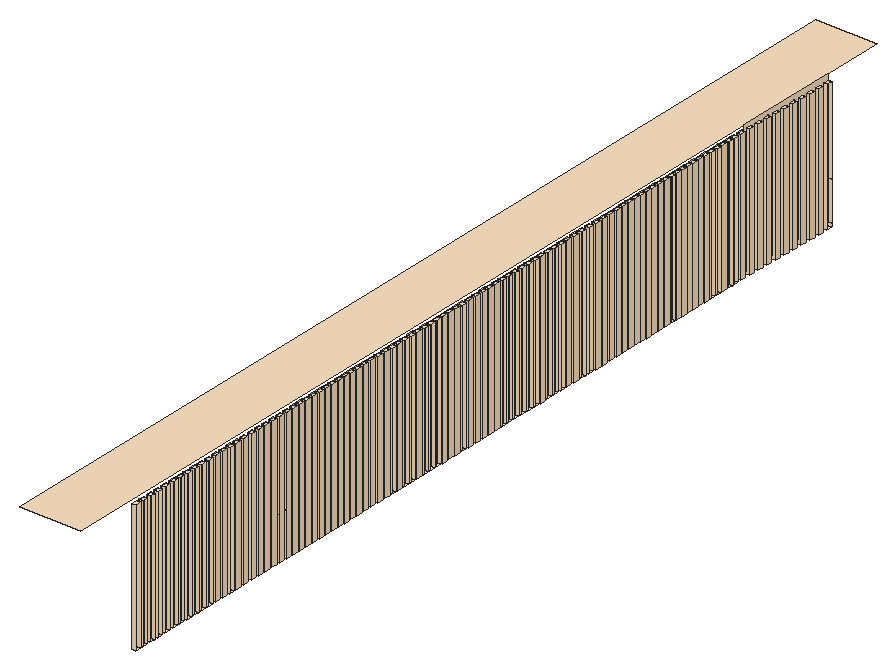
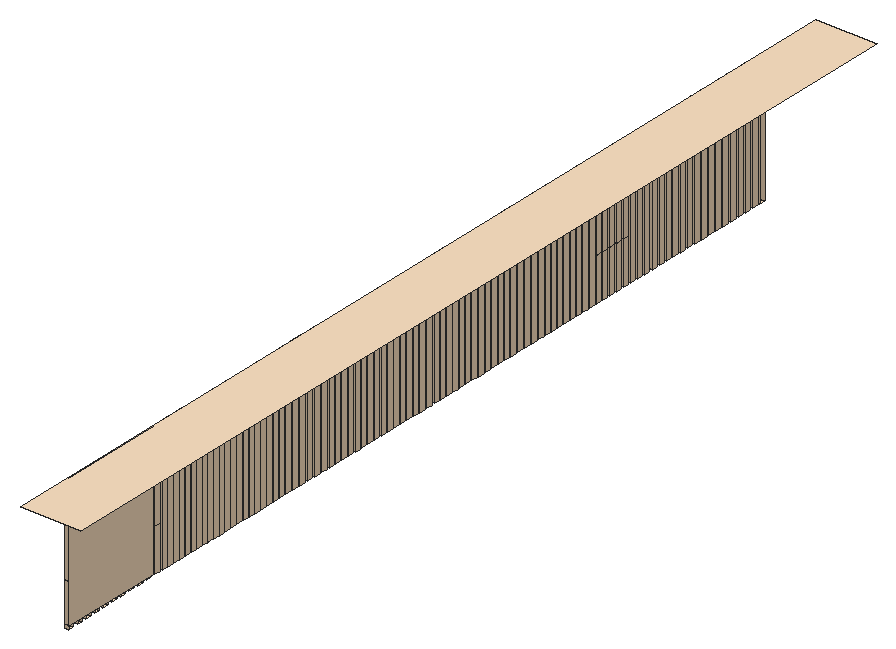
# SketchUp Ruby script. Lengths in inches.
U = 1.inch
M = Sketchup.active_model
def pt(a) = Geom::Point3d.new(a.map { |v| v * U })
def face(e, loops, mat)
  f = e.add_face(loops[0].map { |a| pt(a) })
  loops[1..].each { |l| e.add_face(l.map { |a| pt(a) }).erase! }
  f.material = f.back_material = mat if mat
  f
end
# faces: each face lists its corners as indices into pts; further lists are holes
def faces(e, pts, list, mat = nil) = list.each { |f| face(e, (f[0].is_a?(Array) ? f : [f]).map { |l| l.map { |i| pts[i] } }, mat) }
# xy, xz, yz: faces in a plane at the given z, y or x. An outline is a flat list of corners, or four numbers for a rectangle; further outlines are holes
def ring(l) = l.size == 4 ? [[l[0], l[1]], [l[2], l[1]], [l[2], l[3]], [l[0], l[3]]] : l.each_slice(2).to_a
def flat(e, list, mat, &to3) = list.each { |f| face(e, (f[0].is_a?(Array) ? f : [f]).map { |l| ring(l).map { |u, v| to3.(u, v) } }, mat) }
def xy(e, z, list, mat = nil) = flat(e, list, mat) { |x, y| [x, y, z] }
def xz(e, y, list, mat = nil) = flat(e, list, mat) { |x, z| [x, y, z] }
def yz(e, x, list, mat = nil) = flat(e, list, mat) { |y, z| [x, y, z] }
def lines(e, pts, list) = list.each { |a, b| e.add_line(pt(pts[a]), pt(pts[b])) }
# prism: a flat outline (further loops are holes) pulled along v
def prism(e, loops, v, mat = nil)
  f = face(e, loops, mat); d = Geom::Vector3d.new(v.map { |x| x * U })
  f.pushpull(f.normal.samedirection?(d) ? d.length : -d.length)
end
def box(e, o, s, mat = nil) = prism(e, [[o, [o[0] + s[0], o[1], o[2]], [o[0] + s[0], o[1] + s[1], o[2]], [o[0], o[1] + s[1], o[2]]]], [0, 0, s[2]], mat)
def at(x, y, z, deg = 0) = Geom::Transformation.translation(pt([x, y, z])) * Geom::Transformation.rotation(ORIGIN, Z_AXIS, deg.degrees)
def axes(o, x, y, z) = Geom::Transformation.new([*x, 0, *y, 0, *z, 0, *pt(o).to_a, 1])
def part(name) = M.definitions.add(name)
# library, detail: a bought-in or finely detailed component or shape, given as its bounding box
def library(name, o, s) = part(name).tap { |d| box(d.entities, o, s) }
def detail(e, o, s) = box(e.add_group.entities, o, s)
def put(e, d, t, mat = nil) = e.add_instance(d, t).tap { |i| i.material = mat if mat }
def group(e, t, mat = nil) = e.add_group.tap { |g| g.transformation = t; g.material = mat if mat }.entities
root = M.entities
M.materials.add("[0012_Bisque]").color = [255, 228, 196]
box(root,[9,118.66,100.0625],[0.5625,0.83,19.4375],"[0012_Bisque]")
box(root,[9,119.72,100.0625],[0.5625,0.83,19.4375],"[0012_Bisque]")
box(root,[9,100.09,100.0625],[0.5625,0.83,19.4375],"[0012_Bisque]")
box(root,[9,63.78,100.0625],[0.5625,0.83,19.4375],"[0012_Bisque]")
box(root,[9,126.29,100.0625],[0.5625,0.83,19.4375],"[0012_Bisque]")
box(root,[9,125.29,100.0625],[0.5625,0.83,19.4375],"[0012_Bisque]")
box(root,[9,77.21,100.0625],[0.5625,0.84,19.4375],"[0012_Bisque]")
box(root,[9,81.96,100.0625],[0.5625,0.84,19.4375],"[0012_Bisque]")
box(root,[9,84.28,100.0625],[0.5625,0.83,19.4375],"[0012_Bisque]")
box(root,[9,88.09,100.0625],[0.5625,0.83,19.4375],"[0012_Bisque]")
box(root,[9,86.78,100.0625],[0.5625,0.83,19.4375],"[0012_Bisque]")
box(root,[9,121.97,100.125],[0.5625,0.83,19.375],"[0012_Bisque]")
box(root,[9,106.28,100.125],[0.5625,0.83,19.375],"[0012_Bisque]")
box(root,[9,104.9,100.125],[0.5625,0.83,19.375],"[0012_Bisque]")
box(root,[9,130.47,100.125],[0.5625,0.83,19.375],"[0012_Bisque]")
box(root,[9,127.35,100.125],[0.5625,0.83,19.375],"[0012_Bisque]")
box(root,[9,129.41,100.125],[0.5625,0.83,19.375],"[0012_Bisque]")
box(root,[9,133.72,100.125],[0.5625,0.83,19.375],"[0012_Bisque]")
box(root,[9,120.79,100.125],[0.5625,0.83,19.375],"[0012_Bisque]")
box(root,[9,123.16,100.125],[0.5625,0.83,19.375],"[0012_Bisque]")
box(root,[9,115.29,100.125],[0.5625,0.83,19.375],"[0012_Bisque]")
box(root,[9,89.34,100.125],[0.5625,0.83,19.375],"[0012_Bisque]")
box(root,[9,116.47,100.125],[0.5625,0.83,19.375],"[0012_Bisque]")
box(root,[9,117.6,100.125],[0.5625,0.83,19.375],"[0012_Bisque]")
box(root,[9,66.09,100.125],[0.5625,0.83,19.375],"[0012_Bisque]")
box(root,[9,64.9,100.125],[0.5625,0.83,19.375],"[0012_Bisque]")
box(root,[9,69.96,100.125],[0.5625,0.84,19.375],"[0012_Bisque]")
box(root,[9,68.65,100.125],[0.5625,0.83,19.375],"[0012_Bisque]")
box(root,[9,67.34,100.125],[0.5625,0.83,19.375],"[0012_Bisque]")
box(root,[9,73.59,100.125],[0.5625,0.83,19.375],"[0012_Bisque]")
box(root,[9,43.71,100.125],[0.5625,0.84,19.375],"[0012_Bisque]")
box(root,[9,47.84,100.125],[0.5625,0.83,19.375],"[0012_Bisque]")
box(root,[9,39.9,100.125],[0.5625,0.83,19.375],"[0012_Bisque]")
box(root,[9,46.53,100.125],[0.5625,0.83,19.375],"[0012_Bisque]")
box(root,[9,57.9,100.125],[0.5625,0.83,19.375],"[0012_Bisque]")
box(root,[9,60.28,100.125],[0.5625,0.83,19.375],"[0012_Bisque]")
box(root,[9,61.46,100.125],[0.5625,0.84,19.375],"[0012_Bisque]")
box(root,[9,49.09,100.125],[0.5625,0.83,19.375],"[0012_Bisque]")
box(root,[9,71.28,100.125],[0.5625,0.83,19.375],"[0012_Bisque]")
box(root,[9,41.21,100.125],[0.5625,0.84,19.375],"[0012_Bisque]")
box(root,[9,56.65,100.125],[0.5625,0.83,19.375],"[0012_Bisque]")
box(root,[9,45.09,100.125],[0.5625,0.83,19.375],"[0012_Bisque]")
box(root,[9,59.15,100.125],[0.5625,0.83,19.375],"[0012_Bisque]")
box(root,[9,83.15,100.125],[0.5625,0.83,19.375],"[0012_Bisque]")
box(root,[9,91.71,100.125],[0.5625,0.84,19.375],"[0012_Bisque]")
box(root,[9,128.35,100.125],[0.5625,0.83,19.375],"[0012_Bisque]")
box(root,[9,90.53,100.125],[0.5625,0.83,19.375],"[0012_Bisque]")
box(root,[9,62.65,100.125],[0.5625,0.83,19.375],"[0012_Bisque]")
box(root,[9.0625,110.28,100.0625],[0.5625,0.83,19.4375],"[0012_Bisque]")
box(root,[9.0625,111.53,100.0625],[0.5625,0.83,19.4375],"[0012_Bisque]")
box(root,[9.0625,114.09,100.125],[0.5625,0.83,19.375],"[0012_Bisque]")
box(root,[9.0625,112.84,100.125],[0.5625,0.83,19.375],"[0012_Bisque]")
xy(root,99.78,[[9.03,153.16,9.59,154]],"[0012_Bisque]")
xy(root,99.8125,[[9.02,151.56,9.59,152.4]],"[0012_Bisque]")
xy(root,99.85,[[9.02,149.96,9.58,150.8]],"[0012_Bisque]")
xy(root,99.88,[[9.02,148.37,9.58,149.2]],"[0012_Bisque]")
xy(root,99.92,[[9.02,146.77,9.58,147.6]],"[0012_Bisque]")
xy(root,99.95,[[9.01,145.17,9.58,146]],"[0012_Bisque]")
xy(root,99.99,[[9.01,143.57,9.57,144.4]],"[0012_Bisque]")
xy(root,100.02,[[9.01,141.97,9.57,142.8]],"[0012_Bisque]")
xy(root,100.06,[[9.01,140.37,9.57,141.2]],"[0012_Bisque]")
xy(root,100.09,[[9,138.77,9.57,139.6]],"[0012_Bisque]")
xy(root,100.125,[[9,25.15,9.5625,25.98],[9,26.4,9.5625,27.23],[9,27.78,9.5625,28.61],[9,29.15,9.5625,29.98],[9,30.53,9.5625,31.36],
  [9,32.03,9.5625,32.86],[9,33.28,9.5625,34.11],[9,34.59,9.5625,35.42],[9,35.9,9.5625,36.73],[9,37.21,9.5625,38.05],
  [9,38.53,9.5625,39.36],[9,42.46,9.5625,43.3],[9,50.4,9.5625,51.23],[9,51.71,9.5625,52.55],[9,53.03,9.5625,53.86],
  [9,54.28,9.5625,55.11],[9,55.46,9.5625,56.3],[9,72.46,9.5625,73.3],[9,74.78,9.5625,75.61],[9,76.03,9.5625,76.86],
  [9,78.46,9.5625,79.3],[9,79.65,9.5625,80.48],[9,80.78,9.5625,81.61],[9,85.46,9.5625,86.3],[9,92.9,9.5625,93.73],
  [9,94.03,9.5625,94.86],[9,95.21,9.5625,96.05],[9,96.53,9.5625,97.36],[9,97.78,9.5625,98.61],[9,98.96,9.5625,99.8],
  [9,101.34,9.5625,102.17],[9,102.53,9.5625,103.36],[9,103.78,9.5625,104.61],[9,107.59,9.5625,108.42],[9,108.96,9.5625,109.8],
  [9,124.22,9.5625,125.05],[9,131.54,9.5625,132.37],[9,132.66,9.5625,133.49],[9,134.79,9.5625,135.62],[9,135.85,9.5625,136.68],
  [9,137.17,9.5625,138]],"[0012_Bisque]")
xy(root,119.15,[[9.03,153.16,9.59,154]],"[0012_Bisque]")
xy(root,119.1875,[[9.02,151.56,9.59,152.4]],"[0012_Bisque]")
xy(root,119.22,[[9.02,149.96,9.58,150.8]],"[0012_Bisque]")
xy(root,119.26,[[9.02,148.37,9.58,149.2]],"[0012_Bisque]")
xy(root,119.29,[[9.02,146.77,9.58,147.6]],"[0012_Bisque]")
xy(root,119.33,[[9.01,145.17,9.58,146]],"[0012_Bisque]")
xy(root,119.36,[[9.01,143.57,9.57,144.4]],"[0012_Bisque]")
xy(root,119.4,[[9.01,141.97,9.57,142.8]],"[0012_Bisque]")
xy(root,119.43,[[9.01,140.37,9.57,141.2]],"[0012_Bisque]")
xy(root,119.47,[[9,138.77,9.57,139.6]],"[0012_Bisque]")
xy(root,119.5,[[9,25.15,9.5625,25.98],[9,26.4,9.5625,27.23],[9,27.78,9.5625,28.61],[9,29.15,9.5625,29.98],[9,30.53,9.5625,31.36],
  [9,32.03,9.5625,32.86],[9,33.28,9.5625,34.11],[9,34.59,9.5625,35.42],[9,35.9,9.5625,36.73],[9,37.21,9.5625,38.05],
  [9,38.53,9.5625,39.36],[9,42.46,9.5625,43.3],[9,50.4,9.5625,51.23],[9,51.71,9.5625,52.55],[9,53.03,9.5625,53.86],
  [9,54.28,9.5625,55.11],[9,55.46,9.5625,56.3],[9,72.46,9.5625,73.3],[9,74.78,9.5625,75.61],[9,76.03,9.5625,76.86],
  [9,78.46,9.5625,79.3],[9,79.65,9.5625,80.48],[9,80.78,9.5625,81.61],[9,85.46,9.5625,86.3],[9,92.9,9.5625,93.73],
  [9,94.03,9.5625,94.86],[9,95.21,9.5625,96.05],[9,96.53,9.5625,97.36],[9,97.78,9.5625,98.61],[9,98.96,9.5625,99.8],
  [9,101.34,9.5625,102.17],[9,102.53,9.5625,103.36],[9,103.78,9.5625,104.61],[9,107.59,9.5625,108.42],[9,108.96,9.5625,109.8],
  [9,124.22,9.5625,125.05],[9,131.54,9.5625,132.37],[9,132.66,9.5625,133.49],[9,134.79,9.5625,135.62],[9,135.85,9.5625,136.68],
  [9,137.17,9.5625,138]],"[0012_Bisque]")
xy(root,120,[[9,15.65,9,162.99,0,162.99,0,15.6875]],"[0012_Bisque]")
xz(root,25.15,[[9,100.125,9.5625,119.5]],"[0012_Bisque]")
xz(root,25.98,[[9,100.125,9.5625,119.5]],"[0012_Bisque]")
xz(root,26.4,[[9,100.125,9.5625,119.5]],"[0012_Bisque]")
xz(root,27.23,[[9,100.125,9.5625,119.5]],"[0012_Bisque]")
xz(root,27.78,[[9,100.125,9.5625,119.5]],"[0012_Bisque]")
xz(root,28.61,[[9,100.125,9.5625,119.5]],"[0012_Bisque]")
xz(root,29.15,[[9,100.125,9.5625,119.5]],"[0012_Bisque]")
xz(root,29.98,[[9,100.125,9.5625,119.5]],"[0012_Bisque]")
xz(root,30.53,[[9,100.125,9.5625,119.5]],"[0012_Bisque]")
xz(root,31.36,[[9,100.125,9.5625,119.5]],"[0012_Bisque]")
xz(root,32.03,[[9,100.125,9.5625,119.5]],"[0012_Bisque]")
xz(root,32.86,[[9,100.125,9.5625,119.5]],"[0012_Bisque]")
xz(root,33.28,[[9,100.125,9.5625,119.5]],"[0012_Bisque]")
xz(root,34.11,[[9,100.125,9.5625,119.5]],"[0012_Bisque]")
xz(root,34.59,[[9,100.125,9.5625,119.5]],"[0012_Bisque]")
xz(root,35.42,[[9,100.125,9.5625,119.5]],"[0012_Bisque]")
xz(root,35.9,[[9,100.125,9.5625,119.5]],"[0012_Bisque]")
xz(root,36.73,[[9,100.125,9.5625,119.5]],"[0012_Bisque]")
xz(root,37.21,[[9,100.125,9.5625,119.5]],"[0012_Bisque]")
xz(root,38.05,[[9,100.125,9.5625,119.5]],"[0012_Bisque]")
xz(root,38.53,[[9,100.125,9.5625,119.5]],"[0012_Bisque]")
xz(root,39.36,[[9,100.125,9.5625,119.5]],"[0012_Bisque]")
xz(root,42.46,[[9,100.125,9.5625,119.5]],"[0012_Bisque]")
xz(root,43.3,[[9,100.125,9.5625,119.5]],"[0012_Bisque]")
xz(root,50.4,[[9,100.125,9.5625,106.5],[9,106.5,9.5625,119.5]],"[0012_Bisque]")
xz(root,51.23,[[9,100.125,9.5625,106.5],[9,106.5,9.5625,119.5]],"[0012_Bisque]")
xz(root,51.71,[[9,100.125,9.5625,106.5],[9,106.5,9.5625,119.5]],"[0012_Bisque]")
xz(root,52.55,[[9,100.125,9.5625,106.5],[9,106.5,9.5625,119.5]],"[0012_Bisque]")
xz(root,53.03,[[9,100.125,9.5625,106.5],[9,106.5,9.5625,119.5]],"[0012_Bisque]")
xz(root,53.86,[[9,100.125,9.5625,106.5],[9,106.5,9.5625,119.5]],"[0012_Bisque]")
xz(root,54.28,[[9,100.125,9.5625,106.5],[9,106.5,9.5625,119.5]],"[0012_Bisque]")
xz(root,55.11,[[9,100.125,9.5625,106.5],[9,106.5,9.5625,119.5]],"[0012_Bisque]")
xz(root,55.46,[[9,100.125,9.5625,106.5],[9,106.5,9.5625,119.5]],"[0012_Bisque]")
xz(root,56.3,[[9,100.125,9.5625,106.5],[9,106.5,9.5625,119.5]],"[0012_Bisque]")
xz(root,72.46,[[9,100.125,9.5625,119.5]],"[0012_Bisque]")
xz(root,73.3,[[9,100.125,9.5625,119.5]],"[0012_Bisque]")
xz(root,74.78,[[9,100.125,9.5625,119.5]],"[0012_Bisque]")
xz(root,75.61,[[9,100.125,9.5625,119.5]],"[0012_Bisque]")
xz(root,76.03,[[9,100.125,9.5625,119.5]],"[0012_Bisque]")
xz(root,76.86,[[9,100.125,9.5625,119.5]],"[0012_Bisque]")
xz(root,78.46,[[9,100.125,9.5625,119.5]],"[0012_Bisque]")
xz(root,79.3,[[9,100.125,9.5625,119.5]],"[0012_Bisque]")
xz(root,79.65,[[9,100.125,9.5625,119.5]],"[0012_Bisque]")
xz(root,80.48,[[9,100.125,9.5625,119.5]],"[0012_Bisque]")
xz(root,80.78,[[9,100.125,9.5625,119.5]],"[0012_Bisque]")
xz(root,81.61,[[9,100.125,9.5625,119.5]],"[0012_Bisque]")
xz(root,85.46,[[9,100.125,9.5625,119.5]],"[0012_Bisque]")
xz(root,86.3,[[9,100.125,9.5625,119.5]],"[0012_Bisque]")
xz(root,92.9,[[9,100.125,9.5625,119.5]],"[0012_Bisque]")
xz(root,93.73,[[9,100.125,9.5625,119.5]],"[0012_Bisque]")
xz(root,94.03,[[9,100.125,9.5625,119.5]],"[0012_Bisque]")
xz(root,94.86,[[9,100.125,9.5625,119.5]],"[0012_Bisque]")
xz(root,95.21,[[9,100.125,9.5625,119.5]],"[0012_Bisque]")
xz(root,96.05,[[9,100.125,9.5625,119.5]],"[0012_Bisque]")
xz(root,96.53,[[9,100.125,9.5625,119.5]],"[0012_Bisque]")
xz(root,97.36,[[9,100.125,9.5625,119.5]],"[0012_Bisque]")
xz(root,97.78,[[9,100.125,9.5625,119.5]],"[0012_Bisque]")
xz(root,98.61,[[9,100.125,9.5625,119.5]],"[0012_Bisque]")
xz(root,98.96,[[9,100.125,9.5625,119.5]],"[0012_Bisque]")
xz(root,99.8,[[9,100.125,9.5625,119.5]],"[0012_Bisque]")
xz(root,101.34,[[9,100.125,9.5625,119.5]],"[0012_Bisque]")
xz(root,102.17,[[9,100.125,9.5625,119.5]],"[0012_Bisque]")
xz(root,102.53,[[9,100.125,9.5625,119.5]],"[0012_Bisque]")
xz(root,103.36,[[9,100.125,9.5625,119.5]],"[0012_Bisque]")
xz(root,103.78,[[9,100.125,9.5625,119.5]],"[0012_Bisque]")
xz(root,104.61,[[9,100.125,9.5625,119.5]],"[0012_Bisque]")
xz(root,107.59,[[9,100.125,9.5625,119.5]],"[0012_Bisque]")
xz(root,108.42,[[9,100.125,9.5625,119.5]],"[0012_Bisque]")
xz(root,108.96,[[9,100.125,9.5625,119.5]],"[0012_Bisque]")
xz(root,109.8,[[9,100.125,9.5625,119.5]],"[0012_Bisque]")
xz(root,124.22,[[9,100.125,9.5625,119.5]],"[0012_Bisque]")
xz(root,125.05,[[9,100.125,9.5625,119.5]],"[0012_Bisque]")
xz(root,131.54,[[9,100.125,9.5625,119.5]],"[0012_Bisque]")
xz(root,132.37,[[9,100.125,9.5625,119.5]],"[0012_Bisque]")
xz(root,132.66,[[9,100.125,9.5625,119.5]],"[0012_Bisque]")
xz(root,133.49,[[9,100.125,9.5625,119.5]],"[0012_Bisque]")
xz(root,134.79,[[9,100.125,9.5625,119.5]],"[0012_Bisque]")
xz(root,135.62,[[9,100.125,9.5625,119.5]],"[0012_Bisque]")
xz(root,135.85,[[9,100.125,9.5625,119.5]],"[0012_Bisque]")
xz(root,136.68,[[9,100.125,9.5625,119.5]],"[0012_Bisque]")
xz(root,137.17,[[9,100.125,9.5625,119.5]],"[0012_Bisque]")
xz(root,138,[[9,100.125,9.5625,106.5],[9,106.5,9.5625,119.5]],"[0012_Bisque]")
xz(root,138.77,[[9,100.09,9.57,119.47]],"[0012_Bisque]")
xz(root,139.6,[[9,100.09,9.57,106.47],[9,106.47,9.57,119.47]],"[0012_Bisque]")
xz(root,140.37,[[9.01,100.06,9.57,119.43]],"[0012_Bisque]")
xz(root,141.2,[[9.01,100.06,9.57,106.43],[9.01,106.43,9.57,119.43]],"[0012_Bisque]")
xz(root,141.97,[[9.01,100.02,9.57,119.4]],"[0012_Bisque]")
xz(root,142.8,[[9.01,100.02,9.57,106.4],[9.01,106.4,9.57,119.4]],"[0012_Bisque]")
xz(root,143.57,[[9.01,99.99,9.57,119.36]],"[0012_Bisque]")
xz(root,144.4,[[9.01,99.99,9.57,106.36],[9.01,106.36,9.57,119.36]],"[0012_Bisque]")
xz(root,145.17,[[9.01,99.95,9.58,119.33]],"[0012_Bisque]")
xz(root,146,[[9.01,99.95,9.58,106.33],[9.01,106.33,9.58,119.33]],"[0012_Bisque]")
xz(root,146.77,[[9.02,99.92,9.58,119.29]],"[0012_Bisque]")
xz(root,147.6,[[9.02,99.92,9.58,106.29],[9.02,106.29,9.58,119.29]],"[0012_Bisque]")
xz(root,148.37,[[9.02,99.88,9.58,119.26]],"[0012_Bisque]")
xz(root,149.2,[[9.02,99.88,9.58,106.26],[9.02,106.26,9.58,119.26]],"[0012_Bisque]")
xz(root,149.96,[[9.02,99.85,9.58,119.22]],"[0012_Bisque]")
xz(root,150.8,[[9.02,99.85,9.58,106.22],[9.02,106.22,9.58,119.22]],"[0012_Bisque]")
xz(root,151.56,[[9.02,99.8125,9.59,119.1875]],"[0012_Bisque]")
xz(root,152.4,[[9.02,99.8125,9.59,106.1875],[9.02,106.1875,9.59,119.1875]],"[0012_Bisque]")
xz(root,153.16,[[9.03,99.78,9.59,119.15]],"[0012_Bisque]")
xz(root,154,[[9.03,99.78,9.59,100.32],[9.03,100.32,9.59,106.15],[9.03,106.15,9.59,119.15]],"[0012_Bisque]")
yz(root,9,[[26.4,100.125,27.23,119.5],[27.78,100.125,28.61,119.5],[29.15,100.125,29.98,119.5],[30.53,100.125,31.36,119.5],[32.03,100.125,32.86,119.5],
  [33.28,100.125,34.11,119.5],[34.59,100.125,35.42,119.5],[35.9,100.125,36.73,119.5],[37.21,100.125,38.05,119.5],[38.53,100.125,39.36,119.5],
  [42.46,100.125,43.3,119.5],[50.4,100.125,51.23,106.5],[51.71,100.125,52.55,106.5],[53.03,100.125,53.86,106.5],[54.28,100.125,55.11,106.5],
  [55.46,100.125,56.3,106.5],[72.46,100.125,73.3,119.5],[74.78,100.125,75.61,119.5],[76.03,100.125,76.86,119.5],[78.46,100.125,79.3,119.5],
  [79.65,100.125,80.48,119.5],[80.78,100.125,81.61,119.5],[85.46,100.125,86.3,119.5],[92.9,100.125,93.73,119.5],[94.03,100.125,94.86,119.5],
  [95.21,100.125,96.05,119.5],[96.53,100.125,97.36,119.5],[97.78,100.125,98.61,119.5],[98.96,100.125,99.8,119.5],[101.34,100.125,102.17,119.5],
  [102.53,100.125,103.36,119.5],[103.78,100.125,104.61,119.5],[107.59,100.125,108.42,119.5],[108.96,100.125,109.8,119.5],[124.22,100.125,125.05,119.5],
  [131.54,100.125,132.37,119.5],[132.66,100.125,133.49,119.5],[134.79,100.125,135.62,119.5],[135.85,100.125,136.68,119.5],[137.17,100.125,138,106.5],
  [138.5,100.32,154,120],[50.4,106.5,51.23,119.5],[51.71,106.5,52.55,119.5],[53.03,106.5,53.86,119.5],[54.28,106.5,55.11,119.5],
  [55.46,106.5,56.3,119.5],[137.17,106.5,138,119.5]],"[0012_Bisque]")
yz(root,9.5625,[[50.4,100.125,51.23,119.5],[51.71,100.125,52.55,119.5],[53.03,100.125,53.86,119.5],[54.28,100.125,55.11,119.5],[55.46,100.125,56.3,119.5],
  [137.17,100.125,138,119.5]],"[0012_Bisque]")
yz(root,9.57,[[143.57,99.99,144.4,119.36],[141.97,100.02,142.8,119.4],[140.37,100.06,141.2,119.43],[138.77,100.09,139.6,119.47]],"[0012_Bisque]")
yz(root,9.58,[[149.96,99.85,150.8,119.22],[148.37,99.88,149.2,119.26],[146.77,99.92,147.6,119.29],[145.17,99.95,146,119.33]],"[0012_Bisque]")
yz(root,9.59,[[151.56,99.8125,152.4,119.1875]],"[0012_Bisque]")
